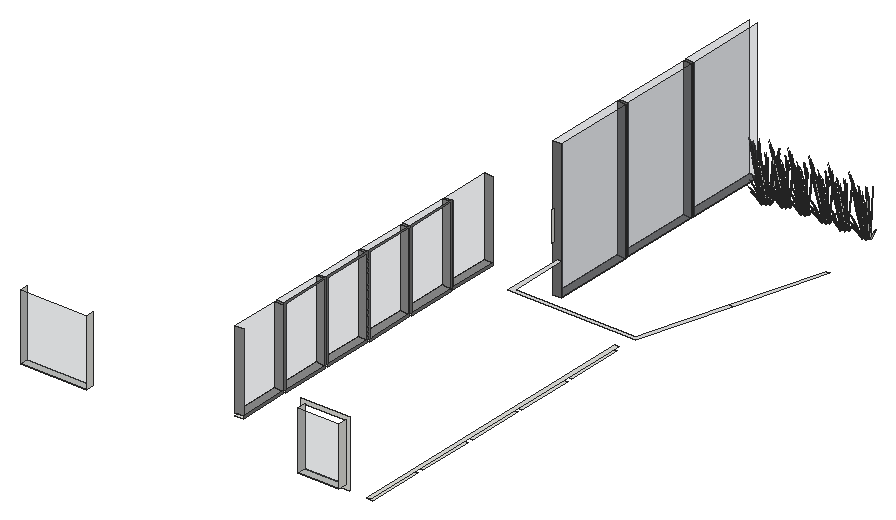
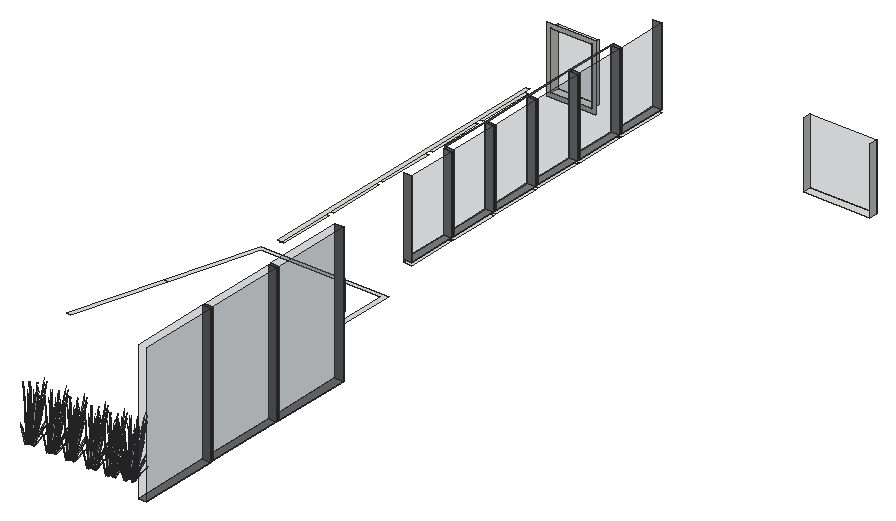
# SketchUp Ruby script. Lengths in inches.
U = 1.inch
M = Sketchup.active_model
def pt(a) = Geom::Point3d.new(a.map { |v| v * U })
def face(e, loops, mat)
  f = e.add_face(loops[0].map { |a| pt(a) })
  loops[1..].each { |l| e.add_face(l.map { |a| pt(a) }).erase! }
  f.material = f.back_material = mat if mat
  f
end
# faces: each face lists its corners as indices into pts; further lists are holes
def faces(e, pts, list, mat = nil) = list.each { |f| face(e, (f[0].is_a?(Array) ? f : [f]).map { |l| l.map { |i| pts[i] } }, mat) }
# xy, xz, yz: faces in a plane at the given z, y or x. An outline is a flat list of corners, or four numbers for a rectangle; further outlines are holes
def ring(l) = l.size == 4 ? [[l[0], l[1]], [l[2], l[1]], [l[2], l[3]], [l[0], l[3]]] : l.each_slice(2).to_a
def flat(e, list, mat, &to3) = list.each { |f| face(e, (f[0].is_a?(Array) ? f : [f]).map { |l| ring(l).map { |u, v| to3.(u, v) } }, mat) }
def xy(e, z, list, mat = nil) = flat(e, list, mat) { |x, y| [x, y, z] }
def xz(e, y, list, mat = nil) = flat(e, list, mat) { |x, z| [x, y, z] }
def yz(e, x, list, mat = nil) = flat(e, list, mat) { |y, z| [x, y, z] }
def lines(e, pts, list) = list.each { |a, b| e.add_line(pt(pts[a]), pt(pts[b])) }
# prism: a flat outline (further loops are holes) pulled along v
def prism(e, loops, v, mat = nil)
  f = face(e, loops, mat); d = Geom::Vector3d.new(v.map { |x| x * U })
  f.pushpull(f.normal.samedirection?(d) ? d.length : -d.length)
end
def box(e, o, s, mat = nil) = prism(e, [[o, [o[0] + s[0], o[1], o[2]], [o[0] + s[0], o[1] + s[1], o[2]], [o[0], o[1] + s[1], o[2]]]], [0, 0, s[2]], mat)
def at(x, y, z, deg = 0) = Geom::Transformation.translation(pt([x, y, z])) * Geom::Transformation.rotation(ORIGIN, Z_AXIS, deg.degrees)
def axes(o, x, y, z) = Geom::Transformation.new([*x, 0, *y, 0, *z, 0, *pt(o).to_a, 1])
def part(name) = M.definitions.add(name)
# library, detail: a bought-in or finely detailed component or shape, given as its bounding box
def library(name, o, s) = part(name).tap { |d| box(d.entities, o, s) }
def detail(e, o, s) = box(e.add_group.entities, o, s)
def put(e, d, t, mat = nil) = e.add_instance(d, t).tap { |i| i.material = mat if mat }
def group(e, t, mat = nil) = e.add_group.tap { |g| g.transformation = t; g.material = mat if mat }.entities
root = M.entities
M.materials.add("Glass_Basic_01").color = [105, 113, 122]
M.materials["Glass_Basic_01"].alpha = 0.25
M.materials.add("LightPink_Translucent").color = [144, 107, 117]
M.materials["LightPink_Translucent"].alpha = 0.75
M.materials.add("M01_Silver_Fog").color = [224, 224, 224]
M.materials.add("M04_Stone_Frost").color = [142, 142, 142]
M.materials.add("M06_Steel_Smoke").color = [114, 114, 114]
c1 = part("blade")
p = [[2.15,0.21,22],[0,0.17,0],[0.09,0.45,0],[2.18,0.31,22],[2.29,0.31,22],[0.38,0.45,0],
  [2.48,0.24,33],[2.49,0.24,33],[2.48,0.22,33]]
faces(c1.entities,p,[[0,1,2,3],[4,5,2,3],[6,3,4,7],[8,0,3,6]])
c2 = part("seeds")
p = [[0.3,-0.1,1.38],[-0.01,-0.03,1.59],[-0.01,-0.03,0.03],[0.14,-0.07,-0.07],[0.29,-0.03,3],[0.15,0.01,3.11]]
faces(c2.entities,p,[[0,1,2,3],[1,0,4,5]],"LightPink_Translucent")
c3 = part("blade with seeds")
put(c3.entities,c1,at(0,0,0))
put(c3.entities,c2,axes([2.4,0.25,30.99],[1.5799,-0.05474,1.17369],[-0.12525,1.92788,0.29478],[-0.07173,-0.02425,1.56792]))
xy(root,403,[[204,295,210,353],[204,355,210,413],[204,415,210,473]],"M06_Steel_Smoke")
xy(root,430,[[300,8,303,49],[300,53,303,94],[300,98,303,139],[300,143,303,184],[300,188,303,229]])
xy(root,432,[[300,6,303,231]])
xy(root,432,[[213,243,305.51,243,324.34,307.35,321.22,307.35,306,255.36,303.26,246,216,246,216,287.79,213,287.79],[321.22,307.35,324.34,307.35,343.2,371.78,340.07,371.78]],"M01_Silver_Fog")
xy(root,435,[[54,0,102,6],[255,0,285,6]])
xy(root,451,[[204,7,210,43],[204,45,210,81],[204,83,210,119],[204,121,210,157],[204,159,210,195],
  [204,197,210,233]])
xy(root,453,[[204,7,210,43],[204,45,210,81],[204,83,210,119],[204,121,210,157],[204,159,210,195],
  [204,197,210,233]],"M04_Stone_Frost")
xz(root,0,[[54,435,102,483],[255,435,285,477]],"Glass_Basic_01")
xz(root,6,[[[252,432,288,480],[255,435,285,477]]])
xz(root,7,[[204,453,210,509]],"M04_Stone_Frost")
xz(root,43,[[204,453,210,509]],"M04_Stone_Frost")
xz(root,45,[[204,453,210,509]],"M04_Stone_Frost")
xz(root,81,[[204,453,210,509]],"M04_Stone_Frost")
xz(root,83,[[204,453,210,509]],"M04_Stone_Frost")
xz(root,119,[[204,453,210,509]],"M04_Stone_Frost")
xz(root,121,[[204,453,210,509]],"M04_Stone_Frost")
xz(root,157,[[204,453,210,509]],"M04_Stone_Frost")
xz(root,159,[[204,453,210,509]],"M04_Stone_Frost")
xz(root,195,[[204,453,210,509]],"M04_Stone_Frost")
xz(root,197,[[204,453,210,509]],"M04_Stone_Frost")
xz(root,233,[[204,453,210,509]],"M04_Stone_Frost")
xz(root,295,[[204,403,210,503]],"M06_Steel_Smoke")
xz(root,353,[[204,403,210,503]],"M06_Steel_Smoke")
xz(root,355,[[204,403,210,503]],"M06_Steel_Smoke")
xz(root,413,[[204,403,210,503]],"M06_Steel_Smoke")
xz(root,415,[[204,403,210,503]],"M06_Steel_Smoke")
yz(root,54,[[0,435,6,483]])
yz(root,102,[[0,435,6,483]])
yz(root,204,[[295,403,353,503],[355,403,413,503],[415,403,473,503],[7,453,43,509],[45,453,81,509],
  [83,453,119,509],[121,453,157,509],[159,453,195,509],[197,453,233,509]],"Glass_Basic_01")
yz(root,210,[[286.46,442.46,288,463.54]])
yz(root,210,[[295,403,353,503],[355,403,413,503],[415,403,473,503]],"Glass_Basic_01")
yz(root,210,[[7,451,43,453],[45,451,81,453],[83,451,119,453],[121,451,157,453],[159,451,195,453],
  [197,451,233,453],[44,453,45,453,45,509,81,509,81,453,82,453,82,510,44,510],[82,453,83,453,83,509,119,509,119,453,120,453,120,510,82,510],[120,453,121,453,121,509,157,509,157,453,158,453,158,510,120,510],[158,453,159,453,159,509,195,509,195,453,196,453,196,510,158,510]],"M06_Steel_Smoke")
yz(root,255,[[0,435,6,477]])
yz(root,285,[[0,435,6,477]])
put(root,c3,axes([228.8,453.28,400.72],[-0.07685,-0.07551,1.74944],[-0.51287,0.04787,-0.27667],[-0.08185,-0.1806,0.14031]))
put(root,c3,axes([231.11,454.21,400.72],[-0.00485,-0.10718,1.74944],[-0.40965,-0.30977,-0.27667],[0.06333,-0.18778,0.14031]))
put(root,c3,axes([231,453.83,400.71],[-0.05103,0.04113,1.77383],[-0.49994,-0.13878,-0.16761],[-0.0181,-0.17951,0.31391]))
put(root,c3,axes([228.28,453.04,400.71],[-0.00937,0.06455,1.77383],[-0.46231,0.23427,-0.16761],[-0.13604,-0.11975,0.31391]))
put(root,c3,axes([228.17,454.18,401.09],[0.55971,-0.13842,0.53763],[0.09714,0.54299,0.4433],[-0.13164,-0.16003,1.11249]))
put(root,c3,axes([229.44,454.28,400.73],[0.4951,0.14079,0.48003],[-0.1693,0.46287,0.3958],[-0.02975,-0.18203,0.9933]))
put(root,c3,axes([229.58,454.45,401.03],[-0.49168,0.25073,-0.1216],[-0.24162,-0.44501,-0.67495],[-0.06487,-0.18753,1.02557]))
put(root,c3,axes([230.6,455.01,401.03],[-0.55221,-0.02668,-0.1216],[0.01509,-0.50521,-0.67495],[0.03836,-0.19458,1.02557]))
put(root,c3,axes([229.57,454.25,400.73],[0.37023,-0.18303,0.0643],[0.18122,0.33376,0.50621],[-0.03575,-0.14712,0.77189]))
put(root,c3,axes([228.3,454.3,400.73],[0.22836,-0.34211,0.0643],[0.3252,0.19918,0.50621],[-0.10513,-0.10968,0.77189]))
put(root,c3,axes([229.43,454.625,401.05],[-0.15148,0.41415,0.35414],[-0.44193,-0.12079,-0.4572],[-0.04052,-0.16674,0.87481]))
put(root,c3,axes([230.5625,454.8,400.73],[0.35779,0.36745,0.48003],[-0.37996,0.3169,0.3958],[0.066,-0.17239,0.9933]))
put(root,c3,axes([228.41,454.26,401.43],[-0.33533,0.51628,-0.13619],[-0.48563,-0.29744,-0.75594],[-0.16881,-0.14586,1.14864]))
put(root,c3,axes([230.7,454.83,400.73],[0.4129,0.02509,0.0643],[-0.01132,0.37891,0.50621],[0.04321,-0.14514,0.77189]))
put(root,c3,axes([230.39,455.09,401.05],[-0.33997,0.28354,0.35414],[-0.32182,-0.32376,-0.4572],[0.04897,-0.1645,0.87481]))
put(root,c3,axes([227.12,454.12,400.72],[-0.10811,-0.0038,1.74944],[-0.34418,0.38014,-0.27667],[-0.18364,-0.07767,0.14031]))
put(root,c3,axes([231.2,456.01,401.03],[-0.46478,-0.29695,-0.1216],[0.26776,-0.43004,-0.67495],[0.13131,-0.14949,1.02557]))
put(root,c3,axes([228.375,454.69,401.05],[0.0776,0.43378,0.35414],[-0.44361,0.11454,-0.4572],[-0.11915,-0.12431,0.87481]))
put(root,c3,axes([227.04,454.98,401.09],[0.41494,-0.39744,0.53763],[0.35786,0.42207,0.4433],[-0.19468,-0.07331,1.11249]))
put(root,c3,axes([232.35,455.88,400.71],[-0.06563,-0.00409,1.77383],[-0.27252,-0.43825,-0.16761],[0.10944,-0.1441,0.31391]))
put(root,c3,axes([227.23,454.97,400.73],[0.0253,-0.40952,0.0643],[0.38204,0.01123,0.50621],[-0.14634,-0.04285,0.77189]))
put(root,c3,axes([230.98,455.97,401.05],[-0.43736,0.07697,0.35414],[-0.11549,-0.43998,-0.4572],[0.12533,-0.11818,0.87481]))
put(root,c3,axes([240.05,457.53,400.72],[-0.07685,-0.07551,1.74944],[-0.51287,0.04787,-0.27667],[-0.08185,-0.1806,0.14031]))
put(root,c3,axes([253.75,457.53,400.72],[-0.07685,-0.07551,1.74944],[-0.51287,0.04787,-0.27667],[-0.08185,-0.1806,0.14031]))
put(root,c3,axes([269,457.53,400.72],[-0.07685,-0.07551,1.74944],[-0.51287,0.04787,-0.27667],[-0.08185,-0.1806,0.14031]))
put(root,c3,axes([282.62,457.53,400.72],[-0.07685,-0.07551,1.74944],[-0.51287,0.04787,-0.27667],[-0.08185,-0.1806,0.14031]))
put(root,c3,axes([298.15,457.53,400.72],[-0.07685,-0.07551,1.74944],[-0.51287,0.04787,-0.27667],[-0.08185,-0.1806,0.14031]))
put(root,c3,axes([231.375,455.9,400.73],[0.34493,0.22649,0.0643],[-0.20082,0.32253,0.50621],[0.11059,-0.10427,0.77189]))
put(root,c3,axes([231.28,455.8,400.73],[0.12461,0.49565,0.48003],[-0.48882,0.08602,0.3958],[0.14406,-0.11657,0.9933]))
put(root,c3,axes([232.6,456.4,400.72],[0.06972,-0.08203,1.74944],[-0.08924,-0.50318,-0.27667],[0.17494,-0.0954,0.14031]))
put(root,c3,axes([226.7,454.4375,400.71],[0.03725,0.05374,1.77383],[-0.17957,0.48312,-0.16761],[-0.18186,0.0035,0.31391]))
put(root,c3,axes([242.35,458.46,400.72],[-0.00485,-0.10718,1.74944],[-0.40965,-0.30977,-0.27667],[0.06333,-0.18778,0.14031]))
put(root,c3,axes([256.06,458.46,400.72],[-0.00485,-0.10718,1.74944],[-0.40965,-0.30977,-0.27667],[0.06333,-0.18778,0.14031]))
put(root,c3,axes([271.31,458.46,400.72],[-0.00485,-0.10718,1.74944],[-0.40965,-0.30977,-0.27667],[0.06333,-0.18778,0.14031]))
put(root,c3,axes([284.92,458.46,400.72],[-0.00485,-0.10718,1.74944],[-0.40965,-0.30977,-0.27667],[0.06333,-0.18778,0.14031]))
put(root,c3,axes([300.45,458.46,400.72],[-0.00485,-0.10718,1.74944],[-0.40965,-0.30977,-0.27667],[0.06333,-0.18778,0.14031]))
put(root,c3,axes([242.24,458.07,400.71],[-0.05103,0.04113,1.77383],[-0.49994,-0.13878,-0.16761],[-0.0181,-0.17951,0.31391]))
put(root,c3,axes([255.95,458.07,400.71],[-0.05103,0.04113,1.77383],[-0.49994,-0.13878,-0.16761],[-0.0181,-0.17951,0.31391]))
put(root,c3,axes([271.2,458.07,400.71],[-0.05103,0.04113,1.77383],[-0.49994,-0.13878,-0.16761],[-0.0181,-0.17951,0.31391]))
put(root,c3,axes([284.81,458.07,400.71],[-0.05103,0.04113,1.77383],[-0.49994,-0.13878,-0.16761],[-0.0181,-0.17951,0.31391]))
put(root,c3,axes([300.34,458.07,400.71],[-0.05103,0.04113,1.77383],[-0.49994,-0.13878,-0.16761],[-0.0181,-0.17951,0.31391]))
put(root,c3,axes([227.49,455.28,401.05],[0.28589,0.33718,0.35414],[-0.32644,0.31919,-0.4572],[-0.16586,-0.04856,0.87481]))
put(root,c3,axes([227.41,455.0625,401.03],[-0.0269,0.54769,-0.1216],[-0.50939,-0.01497,-0.67495],[-0.19618,-0.03804,1.02557]))
put(root,c3,axes([231.22,457.17,401.03],[-0.25281,-0.48765,-0.1216],[0.44869,-0.23964,-0.67495],[0.18908,-0.06434,1.02557]))
put(root,c3,axes([239.52,457.28,400.71],[-0.00937,0.06455,1.77383],[-0.46231,0.23427,-0.16761],[-0.13604,-0.11975,0.31391]))
put(root,c3,axes([253.23,457.28,400.71],[-0.00937,0.06455,1.77383],[-0.46231,0.23427,-0.16761],[-0.13604,-0.11975,0.31391]))
put(root,c3,axes([268.48,457.28,400.71],[-0.00937,0.06455,1.77383],[-0.46231,0.23427,-0.16761],[-0.13604,-0.11975,0.31391]))
put(root,c3,axes([282.09,457.28,400.71],[-0.00937,0.06455,1.77383],[-0.46231,0.23427,-0.16761],[-0.13604,-0.11975,0.31391]))
put(root,c3,axes([297.62,457.28,400.71],[-0.00937,0.06455,1.77383],[-0.46231,0.23427,-0.16761],[-0.13604,-0.11975,0.31391]))
put(root,c3,axes([239.42,458.43,401.09],[0.55971,-0.13842,0.53763],[0.09714,0.54299,0.4433],[-0.13164,-0.16003,1.11249]))
put(root,c3,axes([253.125,458.43,401.09],[0.55971,-0.13842,0.53763],[0.09714,0.54299,0.4433],[-0.13164,-0.16003,1.11249]))
put(root,c3,axes([268.375,458.43,401.09],[0.55971,-0.13842,0.53763],[0.09714,0.54299,0.4433],[-0.13164,-0.16003,1.11249]))
put(root,c3,axes([281.99,458.43,401.09],[0.55971,-0.13842,0.53763],[0.09714,0.54299,0.4433],[-0.13164,-0.16003,1.11249]))
put(root,c3,axes([297.52,458.43,401.09],[0.55971,-0.13842,0.53763],[0.09714,0.54299,0.4433],[-0.13164,-0.16003,1.11249]))
put(root,c3,axes([240.68,458.53,400.73],[0.4951,0.14079,0.48003],[-0.1693,0.46287,0.3958],[-0.02975,-0.18203,0.9933]))
put(root,c3,axes([254.39,458.53,400.73],[0.4951,0.14079,0.48003],[-0.1693,0.46287,0.3958],[-0.02975,-0.18203,0.9933]))
put(root,c3,axes([269.64,458.53,400.73],[0.4951,0.14079,0.48003],[-0.1693,0.46287,0.3958],[-0.02975,-0.18203,0.9933]))
put(root,c3,axes([283.25,458.53,400.73],[0.4951,0.14079,0.48003],[-0.1693,0.46287,0.3958],[-0.02975,-0.18203,0.9933]))
put(root,c3,axes([298.78,458.53,400.73],[0.4951,0.14079,0.48003],[-0.1693,0.46287,0.3958],[-0.02975,-0.18203,0.9933]))
put(root,c3,axes([240.83,458.7,401.03],[-0.49168,0.25073,-0.1216],[-0.24162,-0.44501,-0.67495],[-0.06487,-0.18753,1.02557]))
put(root,c3,axes([254.53,458.7,401.03],[-0.49168,0.25073,-0.1216],[-0.24162,-0.44501,-0.67495],[-0.06487,-0.18753,1.02557]))
put(root,c3,axes([269.78,458.7,401.03],[-0.49168,0.25073,-0.1216],[-0.24162,-0.44501,-0.67495],[-0.06487,-0.18753,1.02557]))
put(root,c3,axes([283.4,458.7,401.03],[-0.49168,0.25073,-0.1216],[-0.24162,-0.44501,-0.67495],[-0.06487,-0.18753,1.02557]))
put(root,c3,axes([298.93,458.7,401.03],[-0.49168,0.25073,-0.1216],[-0.24162,-0.44501,-0.67495],[-0.06487,-0.18753,1.02557]))
put(root,c3,axes([241.85,459.26,401.03],[-0.55221,-0.02668,-0.1216],[0.01509,-0.50521,-0.67495],[0.03836,-0.19458,1.02557]))
put(root,c3,axes([255.56,459.26,401.03],[-0.55221,-0.02668,-0.1216],[0.01509,-0.50521,-0.67495],[0.03836,-0.19458,1.02557]))
put(root,c3,axes([270.8,459.26,401.03],[-0.55221,-0.02668,-0.1216],[0.01509,-0.50521,-0.67495],[0.03836,-0.19458,1.02557]))
put(root,c3,axes([284.42,459.26,401.03],[-0.55221,-0.02668,-0.1216],[0.01509,-0.50521,-0.67495],[0.03836,-0.19458,1.02557]))
put(root,c3,axes([299.95,459.26,401.03],[-0.55221,-0.02668,-0.1216],[0.01509,-0.50521,-0.67495],[0.03836,-0.19458,1.02557]))
put(root,c3,axes([240.82,458.5,400.73],[0.37023,-0.18303,0.0643],[0.18122,0.33376,0.50621],[-0.03575,-0.14712,0.77189]))
put(root,c3,axes([254.52,458.5,400.73],[0.37023,-0.18303,0.0643],[0.18122,0.33376,0.50621],[-0.03575,-0.14712,0.77189]))
put(root,c3,axes([269.77,458.5,400.73],[0.37023,-0.18303,0.0643],[0.18122,0.33376,0.50621],[-0.03575,-0.14712,0.77189]))
put(root,c3,axes([283.39,458.5,400.73],[0.37023,-0.18303,0.0643],[0.18122,0.33376,0.50621],[-0.03575,-0.14712,0.77189]))
put(root,c3,axes([298.92,458.5,400.73],[0.37023,-0.18303,0.0643],[0.18122,0.33376,0.50621],[-0.03575,-0.14712,0.77189]))
put(root,c3,axes([231.05,457.02,401.05],[-0.41757,-0.15024,0.35414],[0.12179,-0.4383,-0.4572],[0.16812,-0.04019,0.87481]))
put(root,c3,axes([226.68,456.22,400.73],[0.14195,-0.49104,0.48003],[0.46669,0.16791,0.3958],[-0.18353,0.02951,0.9933]))
put(root,c3,axes([239.55,458.55,400.73],[0.22836,-0.34211,0.0643],[0.3252,0.19918,0.50621],[-0.10513,-0.10968,0.77189]))
put(root,c3,axes([253.26,458.55,400.73],[0.22836,-0.34211,0.0643],[0.3252,0.19918,0.50621],[-0.10513,-0.10968,0.77189]))
put(root,c3,axes([268.5,458.55,400.73],[0.22836,-0.34211,0.0643],[0.3252,0.19918,0.50621],[-0.10513,-0.10968,0.77189]))
put(root,c3,axes([282.12,458.55,400.73],[0.22836,-0.34211,0.0643],[0.3252,0.19918,0.50621],[-0.10513,-0.10968,0.77189]))
put(root,c3,axes([297.65,458.55,400.73],[0.22836,-0.34211,0.0643],[0.3252,0.19918,0.50621],[-0.10513,-0.10968,0.77189]))
put(root,c3,axes([226.64,456.09,400.73],[-0.18454,-0.3672,0.0643],[0.33652,-0.17973,0.50621],[-0.14834,0.03546,0.77189]))
put(root,c3,axes([240.68,458.87,401.05],[-0.15148,0.41415,0.35414],[-0.44193,-0.12079,-0.4572],[-0.04052,-0.16674,0.87481]))
put(root,c3,axes([254.39,458.87,401.05],[-0.15148,0.41415,0.35414],[-0.44193,-0.12079,-0.4572],[-0.04052,-0.16674,0.87481]))
put(root,c3,axes([269.63,458.87,401.05],[-0.15148,0.41415,0.35414],[-0.44193,-0.12079,-0.4572],[-0.04052,-0.16674,0.87481]))
put(root,c3,axes([283.25,458.87,401.05],[-0.15148,0.41415,0.35414],[-0.44193,-0.12079,-0.4572],[-0.04052,-0.16674,0.87481]))
put(root,c3,axes([298.78,458.87,401.05],[-0.15148,0.41415,0.35414],[-0.44193,-0.12079,-0.4572],[-0.04052,-0.16674,0.87481]))
put(root,c3,axes([241.81,459.05,400.73],[0.35779,0.36745,0.48003],[-0.37996,0.3169,0.3958],[0.066,-0.17239,0.9933]))
put(root,c3,axes([255.52,459.05,400.73],[0.35779,0.36745,0.48003],[-0.37996,0.3169,0.3958],[0.066,-0.17239,0.9933]))
put(root,c3,axes([270.76,459.05,400.73],[0.35779,0.36745,0.48003],[-0.37996,0.3169,0.3958],[0.066,-0.17239,0.9933]))
put(root,c3,axes([284.38,459.05,400.73],[0.35779,0.36745,0.48003],[-0.37996,0.3169,0.3958],[0.066,-0.17239,0.9933]))
put(root,c3,axes([299.91,459.05,400.73],[0.35779,0.36745,0.48003],[-0.37996,0.3169,0.3958],[0.066,-0.17239,0.9933]))
put(root,c3,axes([239.65,458.51,401.43],[-0.33533,0.51628,-0.13619],[-0.48563,-0.29744,-0.75594],[-0.16881,-0.14586,1.14864]))
put(root,c3,axes([253.36,458.51,401.43],[-0.33533,0.51628,-0.13619],[-0.48563,-0.29744,-0.75594],[-0.16881,-0.14586,1.14864]))
put(root,c3,axes([268.61,458.51,401.43],[-0.33533,0.51628,-0.13619],[-0.48563,-0.29744,-0.75594],[-0.16881,-0.14586,1.14864]))
put(root,c3,axes([282.22,458.51,401.43],[-0.33533,0.51628,-0.13619],[-0.48563,-0.29744,-0.75594],[-0.16881,-0.14586,1.14864]))
put(root,c3,axes([297.75,458.51,401.43],[-0.33533,0.51628,-0.13619],[-0.48563,-0.29744,-0.75594],[-0.16881,-0.14586,1.14864]))
put(root,c3,axes([241.94,459.08,400.73],[0.4129,0.02509,0.0643],[-0.01132,0.37891,0.50621],[0.04321,-0.14514,0.77189]))
put(root,c3,axes([255.65,459.08,400.73],[0.4129,0.02509,0.0643],[-0.01132,0.37891,0.50621],[0.04321,-0.14514,0.77189]))
put(root,c3,axes([270.9,459.08,400.73],[0.4129,0.02509,0.0643],[-0.01132,0.37891,0.50621],[0.04321,-0.14514,0.77189]))
put(root,c3,axes([284.51,459.08,400.73],[0.4129,0.02509,0.0643],[-0.01132,0.37891,0.50621],[0.04321,-0.14514,0.77189]))
put(root,c3,axes([300.04,459.08,400.73],[0.4129,0.02509,0.0643],[-0.01132,0.37891,0.50621],[0.04321,-0.14514,0.77189]))
put(root,c3,axes([241.63,459.34,401.05],[-0.33997,0.28354,0.35414],[-0.32182,-0.32376,-0.4572],[0.04897,-0.1645,0.87481]))
put(root,c3,axes([255.34,459.34,401.05],[-0.33997,0.28354,0.35414],[-0.32182,-0.32376,-0.4572],[0.04897,-0.1645,0.87481]))
put(root,c3,axes([270.59,459.34,401.05],[-0.33997,0.28354,0.35414],[-0.32182,-0.32376,-0.4572],[0.04897,-0.1645,0.87481]))
put(root,c3,axes([284.2,459.34,401.05],[-0.33997,0.28354,0.35414],[-0.32182,-0.32376,-0.4572],[0.04897,-0.1645,0.87481]))
put(root,c3,axes([299.73,459.34,401.05],[-0.33997,0.28354,0.35414],[-0.32182,-0.32376,-0.4572],[0.04897,-0.1645,0.87481]))
put(root,c3,axes([238.37,458.36,400.72],[-0.10811,-0.0038,1.74944],[-0.34418,0.38014,-0.27667],[-0.18364,-0.07767,0.14031]))
put(root,c3,axes([252.07,458.36,400.72],[-0.10811,-0.0038,1.74944],[-0.34418,0.38014,-0.27667],[-0.18364,-0.07767,0.14031]))
put(root,c3,axes([267.32,458.36,400.72],[-0.10811,-0.0038,1.74944],[-0.34418,0.38014,-0.27667],[-0.18364,-0.07767,0.14031]))
put(root,c3,axes([280.93,458.36,400.72],[-0.10811,-0.0038,1.74944],[-0.34418,0.38014,-0.27667],[-0.18364,-0.07767,0.14031]))
put(root,c3,axes([296.46,458.36,400.72],[-0.10811,-0.0038,1.74944],[-0.34418,0.38014,-0.27667],[-0.18364,-0.07767,0.14031]))
put(root,c3,axes([242.45,460.25,401.03],[-0.46478,-0.29695,-0.1216],[0.26776,-0.43004,-0.67495],[0.13131,-0.14949,1.02557]))
put(root,c3,axes([256.16,460.25,401.03],[-0.46478,-0.29695,-0.1216],[0.26776,-0.43004,-0.67495],[0.13131,-0.14949,1.02557]))
put(root,c3,axes([271.41,460.25,401.03],[-0.46478,-0.29695,-0.1216],[0.26776,-0.43004,-0.67495],[0.13131,-0.14949,1.02557]))
put(root,c3,axes([285.02,460.25,401.03],[-0.46478,-0.29695,-0.1216],[0.26776,-0.43004,-0.67495],[0.13131,-0.14949,1.02557]))
put(root,c3,axes([300.55,460.25,401.03],[-0.46478,-0.29695,-0.1216],[0.26776,-0.43004,-0.67495],[0.13131,-0.14949,1.02557]))
put(root,c3,axes([231.43,457.16,400.73],[0.18454,0.3672,0.0643],[-0.33652,0.17973,0.50621],[0.14834,-0.03546,0.77189]))
put(root,c3,axes([231.39,457.03,400.73],[-0.14195,0.49104,0.48003],[-0.46669,-0.16791,0.3958],[0.18353,-0.02951,0.9933]))
put(root,c3,axes([227.02,456.22,401.05],[0.41757,0.15024,0.35414],[-0.12179,0.4383,-0.4572],[-0.16812,0.04019,0.87481]))
put(root,c3,axes([239.62,458.94,401.05],[0.0776,0.43378,0.35414],[-0.44361,0.11454,-0.4572],[-0.11915,-0.12431,0.87481]))
put(root,c3,axes([253.33,458.94,401.05],[0.0776,0.43378,0.35414],[-0.44361,0.11454,-0.4572],[-0.11915,-0.12431,0.87481]))
put(root,c3,axes([268.57,458.94,401.05],[0.0776,0.43378,0.35414],[-0.44361,0.11454,-0.4572],[-0.11915,-0.12431,0.87481]))
put(root,c3,axes([282.1875,458.94,401.05],[0.0776,0.43378,0.35414],[-0.44361,0.11454,-0.4572],[-0.11915,-0.12431,0.87481]))
put(root,c3,axes([297.72,458.94,401.05],[0.0776,0.43378,0.35414],[-0.44361,0.11454,-0.4572],[-0.11915,-0.12431,0.87481]))
put(root,c3,axes([238.29,459.22,401.09],[0.41494,-0.39744,0.53763],[0.35786,0.42207,0.4433],[-0.19468,-0.07331,1.11249]))
put(root,c3,axes([251.99,459.22,401.09],[0.41494,-0.39744,0.53763],[0.35786,0.42207,0.4433],[-0.19468,-0.07331,1.11249]))
put(root,c3,axes([267.24,459.22,401.09],[0.41494,-0.39744,0.53763],[0.35786,0.42207,0.4433],[-0.19468,-0.07331,1.11249]))
put(root,c3,axes([280.86,459.22,401.09],[0.41494,-0.39744,0.53763],[0.35786,0.42207,0.4433],[-0.19468,-0.07331,1.11249]))
put(root,c3,axes([296.39,459.22,401.09],[0.41494,-0.39744,0.53763],[0.35786,0.42207,0.4433],[-0.19468,-0.07331,1.11249]))
put(root,c3,axes([243.59,460.125,400.71],[-0.06563,-0.00409,1.77383],[-0.27252,-0.43825,-0.16761],[0.10944,-0.1441,0.31391]))
put(root,c3,axes([257.3,460.125,400.71],[-0.06563,-0.00409,1.77383],[-0.27252,-0.43825,-0.16761],[0.10944,-0.1441,0.31391]))
put(root,c3,axes([272.55,460.125,400.71],[-0.06563,-0.00409,1.77383],[-0.27252,-0.43825,-0.16761],[0.10944,-0.1441,0.31391]))
put(root,c3,axes([286.16,460.125,400.71],[-0.06563,-0.00409,1.77383],[-0.27252,-0.43825,-0.16761],[0.10944,-0.1441,0.31391]))
put(root,c3,axes([301.69,460.125,400.71],[-0.06563,-0.00409,1.77383],[-0.27252,-0.43825,-0.16761],[0.10944,-0.1441,0.31391]))
put(root,c3,axes([238.48,459.22,400.73],[0.0253,-0.40952,0.0643],[0.38204,0.01123,0.50621],[-0.14634,-0.04285,0.77189]))
put(root,c3,axes([252.18,459.22,400.73],[0.0253,-0.40952,0.0643],[0.38204,0.01123,0.50621],[-0.14634,-0.04285,0.77189]))
put(root,c3,axes([267.43,459.22,400.73],[0.0253,-0.40952,0.0643],[0.38204,0.01123,0.50621],[-0.14634,-0.04285,0.77189]))
put(root,c3,axes([281.04,459.22,400.73],[0.0253,-0.40952,0.0643],[0.38204,0.01123,0.50621],[-0.14634,-0.04285,0.77189]))
put(root,c3,axes([296.57,459.22,400.73],[0.0253,-0.40952,0.0643],[0.38204,0.01123,0.50621],[-0.14634,-0.04285,0.77189]))
put(root,c3,axes([232.23,458.62,400.71],[-0.04543,-0.04715,1.77383],[0.09938,-0.50538,-0.16761],[0.17896,-0.03229,0.31391]))
put(root,c3,axes([226.32,456.56,400.72],[-0.08205,0.06992,1.74944],[0.00698,0.51086,-0.27667],[-0.18807,0.06644,0.14031]))
put(root,c3,axes([226.84,456.08,401.03],[0.25281,0.48765,-0.1216],[-0.44869,0.23964,-0.67495],[-0.18908,0.06434,1.02557]))
put(root,c3,axes([230.66,458.18,401.03],[0.0269,-0.54769,-0.1216],[0.50939,0.01497,-0.67495],[0.19618,0.03804,1.02557]))
put(root,c3,axes([242.22,460.21,401.05],[-0.43736,0.07697,0.35414],[-0.11549,-0.43998,-0.4572],[0.12533,-0.11818,0.87481]))
put(root,c3,axes([255.93,460.21,401.05],[-0.43736,0.07697,0.35414],[-0.11549,-0.43998,-0.4572],[0.12533,-0.11818,0.87481]))
put(root,c3,axes([271.18,460.21,401.05],[-0.43736,0.07697,0.35414],[-0.11549,-0.43998,-0.4572],[0.12533,-0.11818,0.87481]))
put(root,c3,axes([284.79,460.21,401.05],[-0.43736,0.07697,0.35414],[-0.11549,-0.43998,-0.4572],[0.12533,-0.11818,0.87481]))
put(root,c3,axes([300.32,460.21,401.05],[-0.43736,0.07697,0.35414],[-0.11549,-0.43998,-0.4572],[0.12533,-0.11818,0.87481]))
put(root,c3,axes([230.58,457.97,401.05],[-0.28589,-0.33718,0.35414],[0.32644,-0.31919,-0.4572],[0.16586,0.04856,0.87481]))
put(root,c3,axes([242.62,460.14,400.73],[0.34493,0.22649,0.0643],[-0.20082,0.32253,0.50621],[0.11059,-0.10427,0.77189]))
put(root,c3,axes([256.33,460.14,400.73],[0.34493,0.22649,0.0643],[-0.20082,0.32253,0.50621],[0.11059,-0.10427,0.77189]))
put(root,c3,axes([271.58,460.14,400.73],[0.34493,0.22649,0.0643],[-0.20082,0.32253,0.50621],[0.11059,-0.10427,0.77189]))
put(root,c3,axes([285.1875,460.14,400.73],[0.34493,0.22649,0.0643],[-0.20082,0.32253,0.50621],[0.11059,-0.10427,0.77189]))
put(root,c3,axes([300.72,460.14,400.73],[0.34493,0.22649,0.0643],[-0.20082,0.32253,0.50621],[0.11059,-0.10427,0.77189]))
put(root,c3,axes([242.52,460.05,400.73],[0.12461,0.49565,0.48003],[-0.48882,0.08602,0.3958],[0.14406,-0.11657,0.9933]))
put(root,c3,axes([256.23,460.05,400.73],[0.12461,0.49565,0.48003],[-0.48882,0.08602,0.3958],[0.14406,-0.11657,0.9933]))
put(root,c3,axes([271.48,460.05,400.73],[0.12461,0.49565,0.48003],[-0.48882,0.08602,0.3958],[0.14406,-0.11657,0.9933]))
put(root,c3,axes([285.09,460.05,400.73],[0.12461,0.49565,0.48003],[-0.48882,0.08602,0.3958],[0.14406,-0.11657,0.9933]))
put(root,c3,axes([300.62,460.05,400.73],[0.12461,0.49565,0.48003],[-0.48882,0.08602,0.3958],[0.14406,-0.11657,0.9933]))
put(root,c3,axes([243.84,460.65,400.72],[0.06972,-0.08203,1.74944],[-0.08924,-0.50318,-0.27667],[0.17494,-0.0954,0.14031]))
put(root,c3,axes([257.55,460.65,400.72],[0.06972,-0.08203,1.74944],[-0.08924,-0.50318,-0.27667],[0.17494,-0.0954,0.14031]))
put(root,c3,axes([272.8,460.65,400.72],[0.06972,-0.08203,1.74944],[-0.08924,-0.50318,-0.27667],[0.17494,-0.0954,0.14031]))
put(root,c3,axes([286.41,460.65,400.72],[0.06972,-0.08203,1.74944],[-0.08924,-0.50318,-0.27667],[0.17494,-0.0954,0.14031]))
put(root,c3,axes([301.94,460.65,400.72],[0.06972,-0.08203,1.74944],[-0.08924,-0.50318,-0.27667],[0.17494,-0.0954,0.14031]))
put(root,c3,axes([231.1,457.85,400.72],[0.10779,-0.00911,1.74944],[0.29564,-0.41839,-0.27667],[0.19172,0.05523,0.14031]))
put(root,c3,axes([226.79,457.44,400.73],[-0.12461,-0.49565,0.48003],[0.48882,-0.08602,0.3958],[-0.14406,0.11657,0.9933]))
put(root,c3,axes([226.69,457.35,400.73],[-0.34493,-0.22649,0.0643],[0.20082,-0.32253,0.50621],[-0.11059,0.10427,0.77189]))
put(root,c3,axes([237.95,458.68,400.71],[0.03725,0.05374,1.77383],[-0.17957,0.48312,-0.16761],[-0.18186,0.0035,0.31391]))
put(root,c3,axes([251.66,458.68,400.71],[0.03725,0.05374,1.77383],[-0.17957,0.48312,-0.16761],[-0.18186,0.0035,0.31391]))
